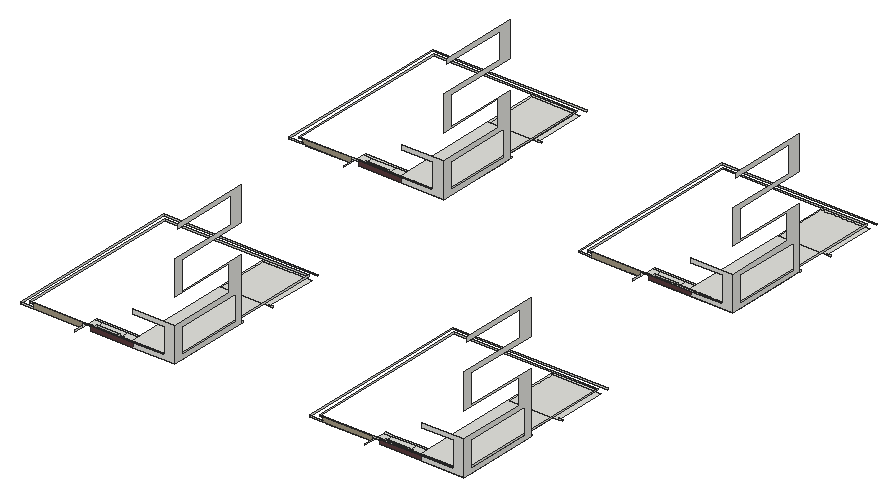
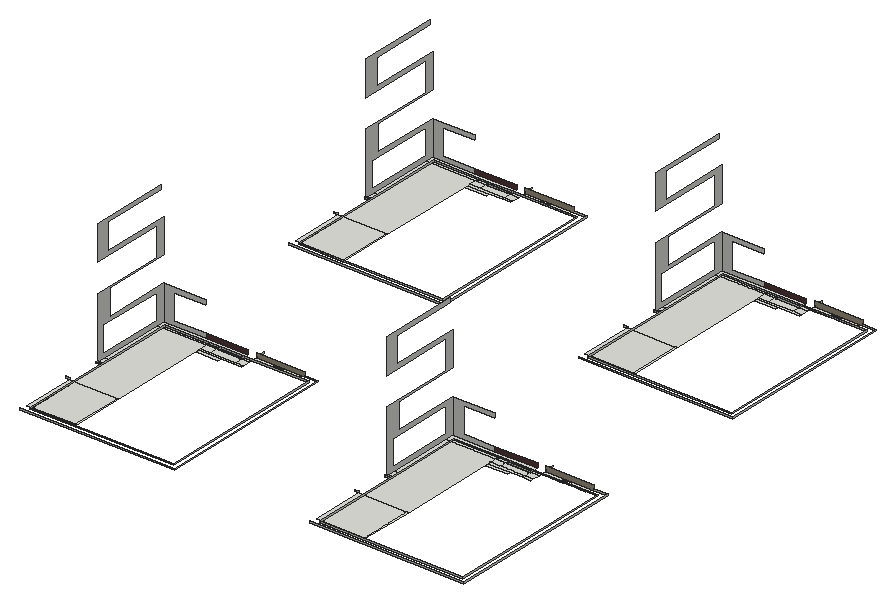
# SketchUp Ruby script. Lengths in inches.
U = 1.inch
M = Sketchup.active_model
def pt(a) = Geom::Point3d.new(a.map { |v| v * U })
def face(e, loops, mat)
  f = e.add_face(loops[0].map { |a| pt(a) })
  loops[1..].each { |l| e.add_face(l.map { |a| pt(a) }).erase! }
  f.material = f.back_material = mat if mat
  f
end
# faces: each face lists its corners as indices into pts; further lists are holes
def faces(e, pts, list, mat = nil) = list.each { |f| face(e, (f[0].is_a?(Array) ? f : [f]).map { |l| l.map { |i| pts[i] } }, mat) }
# xy, xz, yz: faces in a plane at the given z, y or x. An outline is a flat list of corners, or four numbers for a rectangle; further outlines are holes
def ring(l) = l.size == 4 ? [[l[0], l[1]], [l[2], l[1]], [l[2], l[3]], [l[0], l[3]]] : l.each_slice(2).to_a
def flat(e, list, mat, &to3) = list.each { |f| face(e, (f[0].is_a?(Array) ? f : [f]).map { |l| ring(l).map { |u, v| to3.(u, v) } }, mat) }
def xy(e, z, list, mat = nil) = flat(e, list, mat) { |x, y| [x, y, z] }
def xz(e, y, list, mat = nil) = flat(e, list, mat) { |x, z| [x, y, z] }
def yz(e, x, list, mat = nil) = flat(e, list, mat) { |y, z| [x, y, z] }
def lines(e, pts, list) = list.each { |a, b| e.add_line(pt(pts[a]), pt(pts[b])) }
# prism: a flat outline (further loops are holes) pulled along v
def prism(e, loops, v, mat = nil)
  f = face(e, loops, mat); d = Geom::Vector3d.new(v.map { |x| x * U })
  f.pushpull(f.normal.samedirection?(d) ? d.length : -d.length)
end
def box(e, o, s, mat = nil) = prism(e, [[o, [o[0] + s[0], o[1], o[2]], [o[0] + s[0], o[1] + s[1], o[2]], [o[0], o[1] + s[1], o[2]]]], [0, 0, s[2]], mat)
def at(x, y, z, deg = 0) = Geom::Transformation.translation(pt([x, y, z])) * Geom::Transformation.rotation(ORIGIN, Z_AXIS, deg.degrees)
def axes(o, x, y, z) = Geom::Transformation.new([*x, 0, *y, 0, *z, 0, *pt(o).to_a, 1])
def part(name) = M.definitions.add(name)
# library, detail: a bought-in or finely detailed component or shape, given as its bounding box
def library(name, o, s) = part(name).tap { |d| box(d.entities, o, s) }
def detail(e, o, s) = box(e.add_group.entities, o, s)
def put(e, d, t, mat = nil) = e.add_instance(d, t).tap { |i| i.material = mat if mat }
def group(e, t, mat = nil) = e.add_group.tap { |g| g.transformation = t; g.material = mat if mat }.entities
root = M.entities
M.materials.add("[Concrete Tile]").color = [165, 155, 133]
M.materials.add("[Granite Brown]").color = [89, 59, 61]
xy(root,1121.33,[[625.7,1835.1875,715.63,1873.375],[1843.88,1835.1875,1933.82,1873.375],[625.7,3249.875,715.63,3288.0625],[1843.88,3249.875,1933.82,3288.0625]])
xy(root,1134,[[334.58,1799.9375,334.58,1822.9375,404.29,1822.9375,404.29,1806.5625,446.15,1806.5625,446.15,1822.9375,523.04,1822.9375,523.04,1799.9375],[557.88,1799.9375,557.88,1822.9375,890.875,1822.9375,890.875,1835.1875,913.875,1835.1875,913.875,1799.9375],[1552.77,1799.9375,1552.77,1822.9375,1622.48,1822.9375,1622.48,1806.5625,1664.33,1806.5625,1664.33,1822.9375,1741.23,1822.9375,1741.23,1799.9375],[1776.07,1799.9375,1776.07,1822.9375,2109.0625,1822.9375,2109.0625,1835.1875,2132.0625,1835.1875,2132.0625,1799.9375],[431.33,1806.5625,446.15,1822.9375],
  [1649.52,1806.5625,1664.33,1822.9375],[523.04,1822.9375,557.4,1833.75],[653.67,1822.9375,661.4375,1833.75],[661.4375,1822.9375,704.25,1833.75],[704.25,1822.9375,890.875,1835.1875],
  [1741.23,1822.9375,1775.59,1833.75],[1871.86,1822.9375,1879.625,1833.75],[1879.625,1822.9375,1922.4375,1833.75],[1922.4375,1822.9375,2109.0625,1835.1875],[523.04,1833.75,557.4,1865.75],
  [557.88,1833.75,653.67,1835.1875],[653.67,1833.75,661.4375,1835.1875],[661.4375,1833.75,704.25,1835.1875],[1741.23,1833.75,1775.59,1865.75],[1776.07,1833.75,1871.86,1835.1875],
  [1871.86,1833.75,1879.625,1835.1875],[1879.625,1833.75,1922.4375,1835.1875],[557.4,1835.1875,661.4375,1865.75],[661.4375,1835.1875,704.25,1865.75],[704.25,1835.1875,890.875,2295.875],
  [894.3125,1835.1875,913.875,2108.8],[1775.59,1835.1875,1879.625,1865.75],[1879.625,1835.1875,1922.4375,1865.75],[1922.4375,1835.1875,2109.0625,2295.875],[2112.5,1835.1875,2132.0625,2108.8],
  [523.04,1865.75,557.4,1876.125],[557.4,1865.75,661.4375,1876.125],[661.4375,1865.75,704.25,1876.125],[1741.23,1865.75,1775.59,1876.125],[1775.59,1865.75,1879.625,1876.125],
  [1879.625,1865.75,1922.4375,1876.125],[894.3125,2108.8,913.875,2148.83],[2112.5,2108.8,2132.0625,2148.83],[894.3125,2148.83,913.875,2156.01],[2112.5,2148.83,2132.0625,2156.01],
  [704.25,2295.875,710.125,2518.89],[710.125,2295.875,890.875,2518.89],[890.875,2295.875,913.875,2518.89],[1922.4375,2295.875,1928.3125,2518.89],[1928.3125,2295.875,2109.0625,2518.89],
  [2109.0625,2295.875,2132.0625,2518.89],[704.25,2518.89,890.875,2531.375],[1922.4375,2518.89,2109.0625,2531.375],[334.58,3214.625,334.58,3237.625,404.29,3237.625,404.29,3221.25,446.15,3221.25,446.15,3237.625,523.04,3237.625,523.04,3214.625],[557.88,3214.625,557.88,3237.625,890.875,3237.625,890.875,3249.875,913.875,3249.875,913.875,3214.625],
  [1552.77,3214.625,1552.77,3237.625,1622.48,3237.625,1622.48,3221.25,1664.33,3221.25,1664.33,3237.625,1741.23,3237.625,1741.23,3214.625],[1776.07,3214.625,1776.07,3237.625,2109.0625,3237.625,2109.0625,3249.875,2132.0625,3249.875,2132.0625,3214.625],[431.33,3221.25,446.15,3237.625],[1649.52,3221.25,1664.33,3237.625],[523.04,3237.625,557.4,3248.4375],
  [653.67,3237.625,661.4375,3248.4375],[661.4375,3237.625,704.25,3248.4375],[704.25,3237.625,890.875,3249.875],[1741.23,3237.625,1775.59,3248.4375],[1871.86,3237.625,1879.625,3248.4375],
  [1879.625,3237.625,1922.4375,3248.4375],[1922.4375,3237.625,2109.0625,3249.875],[523.04,3248.4375,557.4,3280.4375],[557.88,3248.4375,653.67,3249.875],[653.67,3248.4375,661.4375,3249.875],
  [661.4375,3248.4375,704.25,3249.875],[1741.23,3248.4375,1775.59,3280.4375],[1776.07,3248.4375,1871.86,3249.875],[1871.86,3248.4375,1879.625,3249.875],[1879.625,3248.4375,1922.4375,3249.875],
  [557.4,3249.875,661.4375,3280.4375],[661.4375,3249.875,704.25,3280.4375],[704.25,3249.875,890.875,3710.5625],[894.3125,3249.875,913.875,3523.49],[1775.59,3249.875,1879.625,3280.4375],
  [1879.625,3249.875,1922.4375,3280.4375],[1922.4375,3249.875,2109.0625,3710.5625],[2112.5,3249.875,2132.0625,3523.49],[523.04,3280.4375,557.4,3290.8125],[557.4,3280.4375,661.4375,3290.8125],
  [661.4375,3280.4375,704.25,3290.8125],[1741.23,3280.4375,1775.59,3290.8125],[1775.59,3280.4375,1879.625,3290.8125],[1879.625,3280.4375,1922.4375,3290.8125],[894.3125,3523.49,913.875,3563.51],
  [2112.5,3523.49,2132.0625,3563.51],[894.3125,3563.51,913.875,3570.7],[2112.5,3563.51,2132.0625,3570.7],[704.25,3710.5625,710.125,3933.57],[710.125,3710.5625,890.875,3933.57],
  [890.875,3710.5625,913.875,3933.57],[1922.4375,3710.5625,1928.3125,3933.57],[1928.3125,3710.5625,2109.0625,3933.57],[2109.0625,3710.5625,2132.0625,3933.57],[704.25,3933.57,890.875,3946.0625],
  [1922.4375,3933.57,2109.0625,3946.0625]])
xy(root,1134,[[557.4,1822.9375,557.88,1833.75],[1775.59,1822.9375,1776.07,1833.75],[557.4,1833.75,557.88,1835.1875],[1775.59,1833.75,1776.07,1835.1875],[557.4,3237.625,557.88,3248.4375],
  [1775.59,3237.625,1776.07,3248.4375],[557.4,3248.4375,557.88,3249.875],[1775.59,3248.4375,1776.07,3249.875]],"[Granite Brown]")
xz(root,1799.9375,[[262.875,1134,319.53,1140],[736.96,1134,913.875,1134,913.875,1278.6875,736.96,1278.6875,736.96,1260,869.48,1260,869.48,1152.6875,736.96,1152.6875],[1481.0625,1134,1537.72,1140],[1955.15,1134,2132.0625,1134,2132.0625,1278.6875,1955.15,1278.6875,1955.15,1260,2087.67,1260,2087.67,1152.6875,1955.15,1152.6875]])
xz(root,1799.9375,[[319.53,1134,523.04,1155.4375],[1537.72,1134,1741.23,1155.4375]],"[Concrete Tile]")
xz(root,1799.9375,[[557.88,1134,736.96,1152.6875],[1776.07,1134,1955.15,1152.6875]],"[Granite Brown]")
xz(root,1822.9375,[[285.875,1134,557.4,1140],[557.4,1134,653.67,1140],[653.67,1134,890.875,1140],[1504.0625,1134,1775.59,1140],[1775.59,1134,1871.86,1140],
  [1871.86,1134,2109.0625,1140]])
xz(root,1835.1875,[[557.4,1134,653.67,1140],[1775.59,1134,1871.86,1140]])
xz(root,2148.83,[[894.3125,1134,913.875,1140],[2112.5,1134,2132.0625,1140]])
xz(root,2156.01,[[894.3125,1134,913.875,1140],[2112.5,1134,2132.0625,1140]])
xz(root,2295.875,[[913.875,1134,930.75,1140],[2132.0625,1134,2148.9375,1140]])
xz(root,2531.375,[[285.875,1134,890.875,1140],[1504.0625,1134,2109.0625,1140]])
xz(root,2554.375,[[262.875,1134,913.875,1140],[1481.0625,1134,2132.0625,1140]])
xz(root,3214.625,[[262.875,1134,319.53,1140],[736.96,1134,913.875,1134,913.875,1278.6875,736.96,1278.6875,736.96,1260,869.48,1260,869.48,1152.6875,736.96,1152.6875],[1481.0625,1134,1537.72,1140],[1955.15,1134,2132.0625,1134,2132.0625,1278.6875,1955.15,1278.6875,1955.15,1260,2087.67,1260,2087.67,1152.6875,1955.15,1152.6875]])
xz(root,3214.625,[[319.53,1134,523.04,1155.4375],[1537.72,1134,1741.23,1155.4375]],"[Concrete Tile]")
xz(root,3214.625,[[557.88,1134,736.96,1152.6875],[1776.07,1134,1955.15,1152.6875]],"[Granite Brown]")
xz(root,3237.625,[[285.875,1134,557.4,1140],[557.4,1134,653.67,1140],[653.67,1134,890.875,1140],[1504.0625,1134,1775.59,1140],[1775.59,1134,1871.86,1140],
  [1871.86,1134,2109.0625,1140]])
xz(root,3249.875,[[557.4,1134,653.67,1140],[1775.59,1134,1871.86,1140]])
xz(root,3563.51,[[894.3125,1134,913.875,1140],[2112.5,1134,2132.0625,1140]])
xz(root,3570.7,[[894.3125,1134,913.875,1140],[2112.5,1134,2132.0625,1140]])
xz(root,3710.5625,[[913.875,1134,930.75,1140],[2132.0625,1134,2148.9375,1140]])
xz(root,3946.0625,[[285.875,1134,890.875,1140],[1504.0625,1134,2109.0625,1140]])
xz(root,3969.0625,[[262.875,1134,913.875,1140],[1481.0625,1134,2132.0625,1140]])
yz(root,262.875,[[1799.9375,1134,2554.375,1140],[3214.625,1134,3969.0625,1140]])
yz(root,285.875,[[1822.9375,1134,2531.375,1140],[3237.625,1134,3946.0625,1140]])
yz(root,523.04,[[1763.25,1134,1799.9375,1140],[3177.9375,1134,3214.625,1140]])
yz(root,557.4,[[1822.9375,1134,1835.1875,1140],[3237.625,1134,3249.875,1140]])
yz(root,653.67,[[1822.9375,1134,1835.1875,1140],[3237.625,1134,3249.875,1140]])
yz(root,890.875,[[1822.9375,1134,2531.375,1140],[3237.625,1134,3946.0625,1140]])
yz(root,894.3125,[[2148.83,1134,2156.01,1140],[3563.51,1134,3570.7,1140]])
yz(root,913.875,[[[1799.9375,1134,2148.83,1134,2148.83,1392,1835.1875,1392,1835.1875,1512,2148.83,1512,2148.83,1644,2148.625,1644,2148.625,1656.6875,1814.25,1656.6875,1814.25,1638,2094.15,1638,2094.15,1530.6875,1799.9375,1530.6875,1799.9375,1386,2085.72,1386,2085.72,1278.6875,1799.9375,1278.6875],[1835.1875,1152.6875,2117.96,1260]],[2148.83,1134,2156.01,1140],[[3214.625,1134,3563.51,1134,3563.51,1392,3249.875,1392,3249.875,1512,3563.51,1512,3563.51,1644,3563.3125,1644,3563.3125,1656.6875,3228.9375,1656.6875,3228.9375,1638,3508.84,1638,3508.84,1530.6875,3214.625,1530.6875,3214.625,1386,3500.41,1386,3500.41,1278.6875,3214.625,1278.6875],[3249.875,1152.6875,3532.65,1260]],[3563.51,1134,3570.7,1140]])
yz(root,1481.0625,[[1799.9375,1134,2554.375,1140],[3214.625,1134,3969.0625,1140]])
yz(root,1504.0625,[[1822.9375,1134,2531.375,1140],[3237.625,1134,3946.0625,1140]])
yz(root,1741.23,[[1763.25,1134,1799.9375,1140],[3177.9375,1134,3214.625,1140]])
yz(root,1775.59,[[1822.9375,1134,1835.1875,1140],[3237.625,1134,3249.875,1140]])
yz(root,1871.86,[[1822.9375,1134,1835.1875,1140],[3237.625,1134,3249.875,1140]])
yz(root,2109.0625,[[1822.9375,1134,2531.375,1140],[3237.625,1134,3946.0625,1140]])
yz(root,2112.5,[[2148.83,1134,2156.01,1140],[3563.51,1134,3570.7,1140]])
yz(root,2132.0625,[[[1799.9375,1134,2148.83,1134,2148.83,1392,1835.1875,1392,1835.1875,1512,2148.83,1512,2148.83,1644,2148.625,1644,2148.625,1656.6875,1814.25,1656.6875,1814.25,1638,2094.15,1638,2094.15,1530.6875,1799.9375,1530.6875,1799.9375,1386,2085.72,1386,2085.72,1278.6875,1799.9375,1278.6875],[1835.1875,1152.6875,2117.96,1260]],[2148.83,1134,2156.01,1140],[[3214.625,1134,3563.51,1134,3563.51,1392,3249.875,1392,3249.875,1512,3563.51,1512,3563.51,1644,3563.3125,1644,3563.3125,1656.6875,3228.9375,1656.6875,3228.9375,1638,3508.84,1638,3508.84,1530.6875,3214.625,1530.6875,3214.625,1386,3500.41,1386,3500.41,1278.6875,3214.625,1278.6875],[3249.875,1152.6875,3532.65,1260]],[3563.51,1134,3570.7,1140]])
p = [[2131,2107.15,1133.51],[2132.0625,2148.83,1134],[912.8125,2107.15,1133.51],[913.875,2148.83,1134],[2131,3521.83,1133.51],[2132.0625,3563.51,1134],
  [912.8125,3521.83,1133.51],[913.875,3563.51,1134]]
lines(root,p,[[0,1],[2,3],[4,5],[6,7]])
